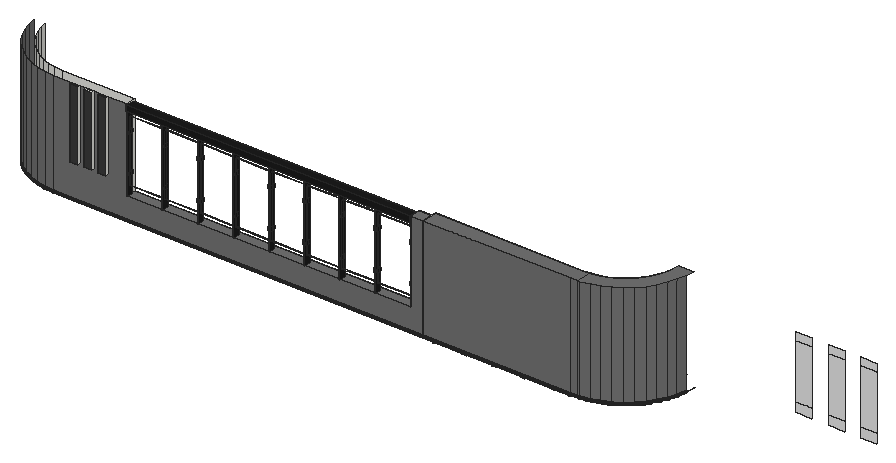
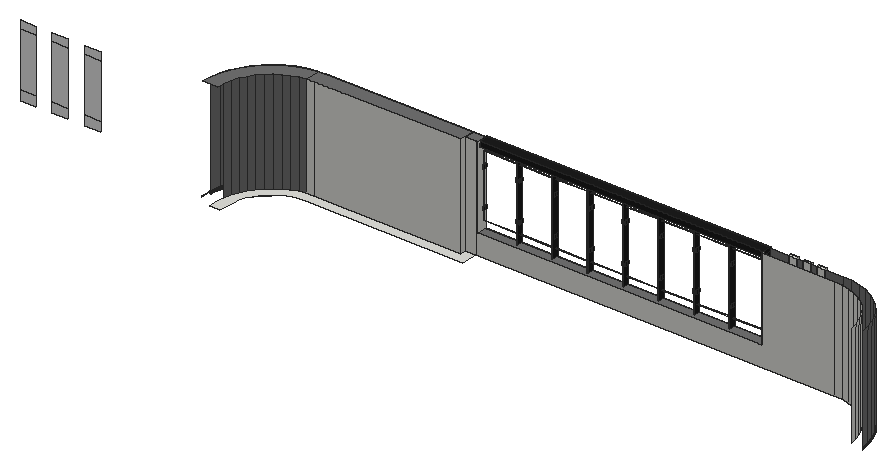
# SketchUp Ruby script. Lengths in inches.
U = 1.inch
M = Sketchup.active_model
def pt(a) = Geom::Point3d.new(a.map { |v| v * U })
def face(e, loops, mat)
  f = e.add_face(loops[0].map { |a| pt(a) })
  loops[1..].each { |l| e.add_face(l.map { |a| pt(a) }).erase! }
  f.material = f.back_material = mat if mat
  f
end
# faces: each face lists its corners as indices into pts; further lists are holes
def faces(e, pts, list, mat = nil) = list.each { |f| face(e, (f[0].is_a?(Array) ? f : [f]).map { |l| l.map { |i| pts[i] } }, mat) }
# xy, xz, yz: faces in a plane at the given z, y or x. An outline is a flat list of corners, or four numbers for a rectangle; further outlines are holes
def ring(l) = l.size == 4 ? [[l[0], l[1]], [l[2], l[1]], [l[2], l[3]], [l[0], l[3]]] : l.each_slice(2).to_a
def flat(e, list, mat, &to3) = list.each { |f| face(e, (f[0].is_a?(Array) ? f : [f]).map { |l| ring(l).map { |u, v| to3.(u, v) } }, mat) }
def xy(e, z, list, mat = nil) = flat(e, list, mat) { |x, y| [x, y, z] }
def xz(e, y, list, mat = nil) = flat(e, list, mat) { |x, z| [x, y, z] }
def yz(e, x, list, mat = nil) = flat(e, list, mat) { |y, z| [x, y, z] }
def lines(e, pts, list) = list.each { |a, b| e.add_line(pt(pts[a]), pt(pts[b])) }
# prism: a flat outline (further loops are holes) pulled along v
def prism(e, loops, v, mat = nil)
  f = face(e, loops, mat); d = Geom::Vector3d.new(v.map { |x| x * U })
  f.pushpull(f.normal.samedirection?(d) ? d.length : -d.length)
end
def box(e, o, s, mat = nil) = prism(e, [[o, [o[0] + s[0], o[1], o[2]], [o[0] + s[0], o[1] + s[1], o[2]], [o[0], o[1] + s[1], o[2]]]], [0, 0, s[2]], mat)
def at(x, y, z, deg = 0) = Geom::Transformation.translation(pt([x, y, z])) * Geom::Transformation.rotation(ORIGIN, Z_AXIS, deg.degrees)
def axes(o, x, y, z) = Geom::Transformation.new([*x, 0, *y, 0, *z, 0, *pt(o).to_a, 1])
def part(name) = M.definitions.add(name)
# library, detail: a bought-in or finely detailed component or shape, given as its bounding box
def library(name, o, s) = part(name).tap { |d| box(d.entities, o, s) }
def detail(e, o, s) = box(e.add_group.entities, o, s)
def put(e, d, t, mat = nil) = e.add_instance(d, t).tap { |i| i.material = mat if mat }
def group(e, t, mat = nil) = e.add_group.tap { |g| g.transformation = t; g.material = mat if mat }.entities
root = M.entities
M.materials.add("[0131_Silver]").color = [28, 28, 28]
M.materials.add("[Color M01]").color = [226, 226, 226]
M.materials.add("[Color M05]").color = [114, 114, 114]
M.materials.add("[Color M07]").color = [58, 58, 58]
M.materials.add("[Translucent_Glass_Blue]").color = [255, 255, 255]
M.materials["[Translucent_Glass_Blue]"].alpha = 0
c1 = part("Group\#11")
xy(c1.entities,0,[[0,0,0.39,2.125]],"[0131_Silver]")
xy(c1.entities,1.5,[[0,0,0.39,2.125]],"[0131_Silver]")
xz(c1.entities,0,[[0,0,0.39,1.5]],"[0131_Silver]")
xz(c1.entities,2.125,[[0,0,0.39,1.5]],"[0131_Silver]")
yz(c1.entities,0,[[0,0,2.125,1.5]],"[0131_Silver]")
yz(c1.entities,0.39,[[0,0,2.125,1.5]],"[0131_Silver]")
c2 = part("Glass railing panel")
xy(c2.entities,0,[[-0.59,0,0,63.98]])
xy(c2.entities,37.71,[[-0.59,0,0,63.98]])
xz(c2.entities,0,[[-0.59,0,0,37.71]])
xz(c2.entities,63.98,[[-0.59,0,0,37.71]])
yz(c2.entities,-0.59,[[0,0,63.98,37.71]])
yz(c2.entities,0,[[0,0,63.98,0,63.98,37.71,0,37.71,0,30.53,1.75,30.53,1.75,28.71,0,28.71],[-0.4,28.71,0,30.53],[0,28.71,1.75,30.53]])
p = [[0,63.98,30.53],[0.39,63.98,30.53]]
lines(c2.entities,p,[[0,1]])
put(c2.entities,c1,axes([0,62.22,28.71],[1,0,0],[0,1.01246,0],[0,0,1.2158]))
put(c2.entities,c1,axes([0,62.22,6.27],[1,0,0],[0,1.01246,0],[0,0,1.2158]))
put(c2.entities,c1,axes([0,0.6,28.71],[1,0,0],[0,1.01246,0],[0,0,1.2158]))
put(c2.entities,c1,axes([0,0.6,6.27],[1,0,0],[0,1.01246,0],[0,0,1.2158]))
put(c2.entities,c1,axes([-0.98,0.6,28.71],[1,0,0],[0,1.01246,0],[0,0,1.2158]))
put(c2.entities,c1,axes([-0.98,62.22,6.27],[1,0,0],[0,1.01246,0],[0,0,1.2158]))
put(c2.entities,c1,axes([-0.98,0.6,6.27],[1,0,0],[0,1.01246,0],[0,0,1.2158]))
put(c2.entities,c1,axes([-0.98,62.22,28.71],[1,0,0],[0,1.01246,0],[0,0,1.2158]))
c3 = part("Group\#1")
xz(c3.entities,0,[[0,0,1.97,38.58]])
xz(c3.entities,1.97,[[0,0,1.97,38.58]])
yz(c3.entities,0,[[0,0,1.97,37.71]])
yz(c3.entities,1.97,[[0,0,1.97,37.71]])
c4 = part("Glass railing section")
xy(c4.entities,37.71,[[2.51,0,3.15,0.39,3.15,0]])
xy(c4.entities,37.71,[[0,0,0.54,520.67],[2.51,0,2.51,63.58,3.15,0.39],[3.15,0.39,2.51,63.58,2.51,520.67,3.15,520.67]],"[0131_Silver]")
xy(c4.entities,38.58,[[0.54,496.0625,2.51,520.67]])
xy(c4.entities,38.58,[[0.54,0,2.51,496.0625]],"[0131_Silver]")
xy(c4.entities,40.46,[[0,0,3.15,520.67]],"[0131_Silver]")
xz(c4.entities,0,[[0,37.71,0.54,37.71,0.54,38.58,2.51,38.58,2.51,37.71,3.15,37.71,3.15,40.46,0,40.46]],"[0131_Silver]")
xz(c4.entities,520.67,[[0,37.71,0,40.46,3.15,40.46,3.15,37.71,2.51,37.71,2.51,38.58,0.54,38.58,0.54,37.71]])
yz(c4.entities,0,[[0,37.71,520.67,40.46]],"[0131_Silver]")
yz(c4.entities,0.54,[[496.0625,37.71,520.67,38.58]])
yz(c4.entities,0.54,[[0,37.71,496.0625,38.58]],"[0131_Silver]")
yz(c4.entities,2.51,[[0,37.71,496.0625,38.58],[496.0625,37.71,520.67,38.58]])
yz(c4.entities,3.15,[[0,37.71,520.67,40.46]],"[0131_Silver]")
put(c4.entities,c2,axes([1.8,65.35,3.9375],[1,0,0],[0,0.98769,0],[0,0,0.8225]),"[Translucent_Glass_Blue]")
put(c4.entities,c2,axes([1.8,130.31,3.9375],[1,0,0],[0,0.98769,0],[0,0,0.8225]),"[Translucent_Glass_Blue]")
put(c4.entities,c2,axes([1.8,195.28,3.9375],[1,0,0],[0,0.98769,0],[0,0,0.8225]),"[Translucent_Glass_Blue]")
put(c4.entities,c2,axes([1.8,260.24,3.9375],[1,0,0],[0,0.98769,0],[0,0,0.8225]),"[Translucent_Glass_Blue]")
put(c4.entities,c2,axes([1.8,325.2,3.9375],[1,0,0],[0,0.98769,0],[0,0,0.8225]),"[Translucent_Glass_Blue]")
put(c4.entities,c2,axes([1.8,390.16,3.9375],[1,0,0],[0,0.98769,0],[0,0,0.8225]),"[Translucent_Glass_Blue]")
put(c4.entities,c2,axes([1.8,455.12,3.9375],[1,0,0],[0,0.98769,0],[0,0,0.8225]),"[Translucent_Glass_Blue]")
put(c4.entities,c2,axes([1.8,0.39,3.9375],[1,0,0],[0,0.98769,0],[0,0,0.8225]),"[Translucent_Glass_Blue]")
put(c4.entities,c3,at(0.54,128.9375,0),"[0131_Silver]")
g1 = group(c4.entities,at(0.54,63.98,0),"[0131_Silver]")
xz(g1,0,[[0,0,1.97,38.58]])
xz(g1,1.97,[[0,0,1.97,38.58]])
yz(g1,0,[[0,0,1.97,37.71]])
yz(g1,1.97,[[0,0,1.97,37.71]])
put(c4.entities,c3,at(0.54,193.9,0),"[0131_Silver]")
put(c4.entities,c3,at(0.54,258.86,0),"[0131_Silver]")
put(c4.entities,c3,at(0.54,323.82,0),"[0131_Silver]")
put(c4.entities,c3,at(0.54,388.78,0),"[0131_Silver]")
put(c4.entities,c3,at(0.54,453.74,0),"[0131_Silver]")
put(c4.entities,c3,at(0.54,518.7,0),"[0131_Silver]")
c5 = part("Glass+Railing")
put(c5.entities,c4,axes([0,0,0],[1,0,0],[0,0.95652,0],[0,0,1]),"[0131_Silver]")
xy(root,251.12,[[157.86,0.53,159.39,0.93],[168.11,0.53,169.64,0.93],[178.36,0.53,179.89,0.93],[188.61,0.53,190.14,0.93],[198.86,0.53,200.39,0.93]])
xy(root,252,[[150.375,4.65,154.02,4.65,154.02,6.39,205.875,6.39,208.3,6.55,210.69,7.03,213,7.81,215.18,8.88,217.2,10.24,219.03,11.84,220.64,13.67,221.99,15.7,223.07,17.88,223.85,20.18,224.32,22.57,224.48,25,224.48,28.65,221.07,28.65,220.7,23.05,220.32,21.13,219.69,19.28,218.83,17.52,217.74,15.9,216.45,14.42,214.98,13.13,213.35,12.05,211.6,11.18,209.75,10.55,207.83,10.17,205.76,10.04,150.375,10.04]])
xy(root,259.1875,[[49.81,1,149.56,4.65]],"[Color M05]")
xy(root,263.625,[[30.59,0,33.34,1],[35.53,0,38.28,1],[40.47,0,43.22,1]])
xy(root,288,[[30.59,0,33.34,1],[35.53,0,38.28,1],[40.47,0,43.22,1]])
xy(root,288,[[149.56,1,154.02,4.65],[154.02,1,205.875,1,208.3,1.16,208.3,6.55,205.875,6.39,154.02,6.39],[208.3,1.16,209.01,1.21,212.09,1.82,215.06,2.83,217.875,4.22,220.49,5.96,222.85,8.03,224.92,10.39,226.66,13,228.05,15.82,229.06,18.79,229.67,21.87,229.875,25,224.48,25,224.32,22.57,223.85,20.18,223.07,17.88,221.99,15.7,220.64,13.67,219.03,11.84,217.2,10.24,215.18,8.88,213,7.81,210.69,7.03,208.3,6.55]],"[Color M05]")
xz(root,0,[[30.59,263.625,33.34,288],[35.53,263.625,38.28,288],[40.47,263.625,43.22,288]],"[Color M07]")
xz(root,1,[[30.59,263.625,33.34,288],[35.53,263.625,38.28,288],[40.47,263.625,43.22,288]])
xz(root,1,[[24.25,252,154.02,252,154.02,288,149.56,288,149.56,259.1875,49.81,259.1875,49.81,288,43.22,288,43.22,263.625,40.47,263.625,40.47,288,38.28,288,38.28,263.625,35.53,263.625,35.53,288,33.34,288,33.34,263.625,30.59,263.625,30.59,288,24.25,288],[154.02,252,205.875,288]],"[Color M05]")
xz(root,4.65,[[24.37,252,24.37,288,49.81,288,49.81,259.1875,149.56,259.1875,149.56,288,150.375,288,150.375,252],[150.375,252,154.02,288]])
xz(root,6.39,[[154.02,252,205.875,288]])
xz(root,23,[[267.39,257.79,273.02,261.06],[279.08,257.79,284.71,261.06],[290.02,257.79,295.64,261.06],[267.39,261.06,273.02,280.31],[279.08,261.06,284.71,280.31],
  [290.02,261.06,295.64,280.31],[267.39,280.31,273.02,283.04],[279.08,280.31,284.71,283.04],[290.02,280.31,295.64,283.04]],"[Color M01]")
yz(root,30.59,[[0,263.625,1,288]])
yz(root,33.34,[[0,263.625,1,288]])
yz(root,35.53,[[0,263.625,1,288]])
yz(root,38.28,[[0,263.625,1,288]])
yz(root,40.47,[[0,263.625,1,288]])
yz(root,43.22,[[0,263.625,1,288]])
yz(root,49.81,[[1,259.1875,4.65,288]])
yz(root,149.56,[[1,259.1875,4.65,288]])
yz(root,154.02,[[1,252,4.65,288],[4.65,252,6.39,288]])
p = [[21.1,1.07,251.1875],[21.11,1.13,251.12],[24.25,0.93,251.12],[24.25,0.87,251.1875],[21.12,1.21,251.0625],[24.25,1,251.0625],
  [154.02,0.93,251.12],[157.86,0.93,251.12],[159.39,0.93,251.12],[168.11,0.93,251.12],[169.64,0.93,251.12],[178.36,0.93,251.12],
  [179.89,0.93,251.12],[188.61,0.93,251.12],[190.14,0.93,251.12],[198.86,0.93,251.12],[200.39,0.93,251.12],[205.88,0.93,251.12],
  [205.88,0.87,251.1875],[154.02,0.87,251.1875],[154.02,1,251.0625],[205.875,1,251.0625],[208.31,1.09,251.12],[209.02,1.13,251.12],
  [209.03,1.07,251.1875],[208.3125,1.03,251.1875],[208.3,1.16,251.0625],[209.01,1.21,251.0625],[18,1.6875,251.1875],[18.02,1.75,251.12],
  [18.04,1.82,251.0625],[212.11,1.75,251.12],[212.12,1.6875,251.1875],[212.09,1.82,251.0625],[15.01,2.7,251.1875],[15.04,2.76,251.12],
  [15.07,2.83,251.0625],[215.09,2.76,251.12],[215.11,2.7,251.1875],[215.06,2.83,251.0625],[12.18,4.1,251.1875],[12.21,4.15,251.12],
  [217.91,4.15,251.12],[217.94,4.1,251.1875],[12.25,4.22,251.0625],[217.875,4.22,251.0625],[9.56,5.85,251.1875],[9.6,5.9,251.12],
  [220.53,5.9,251.12],[220.57,5.85,251.1875],[9.64,5.96,251.0625],[220.49,5.96,251.0625],[7.18,7.93,251.1875],[7.23,7.98,251.12],
  [7.28,8.03,251.0625],[222.9,7.98,251.12],[222.94,7.93,251.1875],[222.85,8.03,251.0625],[5.1,10.31,251.1875],[5.15,10.35,251.12],
  [224.97,10.35,251.12],[225.02,10.31,251.1875],[5.21,10.39,251.0625],[224.92,10.39,251.0625],[3.35,12.93,251.1875],[3.4,12.96,251.12],
  [3.47,13,251.0625],[226.66,13,251.0625],[226.72,12.96,251.12],[226.78,12.93,251.1875],[1.95,15.76,251.1875],[2.01,15.79,251.12],
  [228.11,15.79,251.12],[228.17,15.76,251.1875],[2.08,15.82,251.0625],[228.05,15.82,251.0625],[0.9375,18.75,251.1875],[1,18.77,251.12],
  [1.07,18.79,251.0625],[229.06,18.79,251.0625],[229.125,18.77,251.12],[229.1875,18.75,251.1875],[0.32,21.85,251.1875],[0.38,21.86,251.12],
  [0.46,21.87,251.0625],[229.74,21.86,251.12],[229.8,21.85,251.1875],[229.67,21.87,251.0625],[21.09,1.02,251.27],[24.24,0.82,251.27],
  [205.88,0.82,251.27],[154.02,0.82,251.27],[209.03,1.02,251.27],[208.32,0.98,251.27],[17.99,1.64,251.27],[212.13,1.64,251.27],
  [15,2.66,251.27],[215.13,2.66,251.27],[12.16,4.06,251.27],[217.97,4.06,251.27],[9.53,5.8125,251.27],[220.6,5.8125,251.27],
  [7.15,7.9,251.27],[222.98,7.9,251.27],[5.0625,10.28,251.27],[225.0625,10.28,251.27],[3.31,12.91,251.27],[226.82,12.91,251.27],
  [1.91,15.75,251.27],[228.22,15.75,251.27],[0.89,18.74,251.27],[229.23,18.74,251.27],[0.27,21.84,251.27],[229.85,21.84,251.27],
  [21.09,0.99,251.35],[24.24,0.78,251.35],[205.88,0.78,251.35],[154.02,0.78,251.35],[209.04,0.99,251.35],[208.32,0.94,251.35],
  [17.98,1.6,251.35],[212.14,1.6,251.35],[14.98,2.625,251.35],[215.14,2.625,251.35],[12.14,4.02,251.35],[217.99,4.02,251.35],
  [9.51,5.78,251.35],[220.62,5.78,251.35],[7.125,7.875,251.35],[223,7.875,251.35],[5.03,10.26,251.35],[225.09,10.26,251.35],
  [3.27,12.89,251.35],[226.85,12.89,251.35],[1.875,15.73,251.35],[228.25,15.73,251.35],[0.85,18.73,251.35],[229.27,18.73,251.35],
  [0.24,21.84,251.35],[229.89,21.84,251.35],[21.08,0.96,251.53],[21.09,0.96,251.4375],[24.24,0.76,251.4375],[24.24,0.75,251.53],
  [154.02,0.76,251.4375],[205.88,0.76,251.4375],[205.88,0.75,251.53],[154.02,0.75,251.53],[208.32,0.92,251.4375],[209.04,0.96,251.4375],
  [209.04,0.96,251.53],[208.32,0.91,251.53],[17.97,1.58,251.53],[17.98,1.58,251.4375],[212.15,1.58,251.4375],[212.15,1.58,251.53],
  [14.97,2.6,251.53],[14.97,2.6,251.4375],[215.15,2.6,251.4375],[215.16,2.6,251.53],[12.125,4,251.53],[12.13,4,251.4375],
  [218,4,251.4375],[218,4,251.53],[9.49,5.76,251.53],[9.49,5.77,251.4375],[220.63,5.77,251.4375],[220.64,5.76,251.53],
  [7.1,7.85,251.53],[7.11,7.86,251.4375],[223.02,7.86,251.4375],[223.02,7.85,251.53],[5.01,10.24,251.53],[5.02,10.24,251.4375],
  [225.11,10.24,251.4375],[225.11,10.24,251.53],[3.25,12.875,251.53],[3.25,12.88,251.4375],[226.87,12.88,251.4375],[226.875,12.875,251.53],
  [1.85,15.72,251.53],[1.85,15.72,251.4375],[228.27,15.72,251.4375],[228.28,15.72,251.53],[0.83,18.72,251.53],[0.83,18.73,251.4375],
  [229.29,18.73,251.4375],[229.3,18.72,251.53],[0.21,21.83,251.53],[0.21,21.84,251.4375],[229.91,21.84,251.4375],[229.92,21.83,251.53],
  [230.12,24.98,251.4375],[230.125,24.98,251.53],[21.09,0.96,251.625],[24.24,0.76,251.625],[205.88,0.76,251.625],[154.02,0.76,251.625],
  [209.04,0.96,251.625],[208.32,0.92,251.625],[17.98,1.58,251.625],[212.15,1.58,251.625],[14.97,2.6,251.625],[215.15,2.6,251.625],
  [12.13,4,251.625],[218,4,251.625],[9.49,5.77,251.625],[220.63,5.77,251.625],[7.11,7.86,251.625],[223.02,7.86,251.625],
  [5.02,10.24,251.625],[225.11,10.24,251.625],[3.25,12.88,251.625],[226.87,12.88,251.625],[1.85,15.72,251.625],[228.27,15.72,251.625],
  [0.83,18.73,251.625],[229.29,18.73,251.625],[0.21,21.84,251.625],[229.91,21.84,251.625],[230.12,24.98,251.625],[21.09,0.99,251.71],
  [24.24,0.78,251.71],[205.88,0.78,251.71],[154.02,0.78,251.71],[209.04,0.99,251.71],[208.32,0.94,251.71],[17.98,1.6,251.71],
  [212.14,1.6,251.71],[14.98,2.625,251.71],[215.14,2.625,251.71],[12.14,4.02,251.71],[217.99,4.02,251.71],[9.51,5.78,251.71],
  [220.62,5.78,251.71],[7.125,7.875,251.71],[223,7.875,251.71],[5.03,10.26,251.71],[225.09,10.26,251.71],[3.27,12.89,251.71],
  [226.85,12.89,251.71],[1.875,15.73,251.71],[228.25,15.73,251.71],[0.85,18.73,251.71],[229.27,18.73,251.71],[0.24,21.84,251.71],
  [229.89,21.84,251.71],[21.09,1.02,251.8],[24.24,0.82,251.8],[205.88,0.82,251.8],[154.02,0.82,251.8],[209.03,1.02,251.8],
  [208.32,0.98,251.8],[17.99,1.64,251.8],[212.13,1.64,251.8],[15,2.66,251.8],[215.13,2.66,251.8],[12.16,4.06,251.8],
  [217.97,4.06,251.8],[9.53,5.8125,251.8],[220.6,5.8125,251.8],[7.15,7.9,251.8],[222.98,7.9,251.8],[5.0625,10.28,251.8],
  [225.0625,10.28,251.8],[3.31,12.91,251.8],[226.82,12.91,251.8],[1.91,15.75,251.8],[228.22,15.75,251.8],[0.89,18.74,251.8],
  [229.23,18.74,251.8],[0.27,21.84,251.8],[229.85,21.84,251.8],[21.1,1.07,251.875],[24.25,0.87,251.875],[205.88,0.87,251.875],
  [154.02,0.87,251.875],[209.03,1.07,251.875],[208.3125,1.03,251.875],[18,1.6875,251.875],[212.12,1.6875,251.875],[15.01,2.7,251.875],
  [215.11,2.7,251.875],[12.18,4.1,251.875],[217.94,4.1,251.875],[9.56,5.85,251.875],[220.57,5.85,251.875],[7.18,7.93,251.875],
  [222.94,7.93,251.875],[5.1,10.31,251.875],[225.02,10.31,251.875],[3.35,12.93,251.875],[226.78,12.93,251.875],[1.95,15.76,251.875],
  [228.17,15.76,251.875],[0.9375,18.75,251.875],[229.1875,18.75,251.875],[0.32,21.85,251.875],[229.8,21.85,251.875],[21.11,1.13,251.94],
  [24.25,0.93,251.94],[21.12,1.21,252],[24.25,1,252],[205.88,0.93,251.94],[154.02,0.93,251.94],[205.875,1,252],
  [154.02,1,252],[209.02,1.13,251.94],[208.31,1.09,251.94],[209.01,1.21,252],[208.3,1.16,252],[18.02,1.75,251.94],
  [18.04,1.82,252],[212.11,1.75,251.94],[212.09,1.82,252],[15.04,2.76,251.94],[15.07,2.83,252],[215.09,2.76,251.94],
  [215.06,2.83,252],[12.21,4.15,251.94],[217.91,4.15,251.94],[12.25,4.22,252],[217.875,4.22,252],[9.6,5.9,251.94],
  [220.53,5.9,251.94],[9.64,5.96,252],[220.49,5.96,252],[7.23,7.98,251.94],[7.28,8.03,252],[222.9,7.98,251.94],
  [222.85,8.03,252],[5.15,10.35,251.94],[224.97,10.35,251.94],[5.21,10.39,252],[224.92,10.39,252],[3.4,12.96,251.94],
  [3.47,13,252],[226.72,12.96,251.94],[226.66,13,252],[2.01,15.79,251.94],[228.11,15.79,251.94],[2.08,15.82,252],
  [228.05,15.82,252],[1,18.77,251.94],[1.07,18.79,252],[229.125,18.77,251.94],[229.06,18.79,252],[0.38,21.86,251.94],
  [0.46,21.87,252],[229.74,21.86,251.94],[229.67,21.87,252],[24.25,1,288],[21.12,1.21,288],[208.3,1.16,288],
  [205.875,1,288],[18.04,1.82,288],[209.01,1.21,288],[212.09,1.82,288],[15.07,2.83,288],[215.06,2.83,288],
  [12.25,4.22,288],[217.875,4.22,288],[9.64,5.96,288],[220.49,5.96,288],[24.37,4.65,252],[21.59,4.83,252],
  [21.59,4.83,288],[24.37,4.65,288],[18.98,5.35,252],[18.98,5.35,288],[16.46,6.2,252],[16.46,6.2,288],
  [7.28,8.03,288],[222.85,8.03,288],[14.08,7.38,252],[14.08,7.38,288],[208.3,6.55,252],[205.875,6.39,252],
  [205.875,6.39,288],[208.3,6.55,288],[210.69,7.03,252],[210.69,7.03,288],[213,7.81,252],[213,7.81,288],
  [11.86,8.86,252],[11.86,8.86,288],[215.18,8.88,252],[215.18,8.88,288],[5.21,10.39,288],[224.92,10.39,288],
  [9.86,10.61,252],[9.86,10.61,288],[217.2,10.24,252],[217.2,10.24,288],[219.03,11.84,252],[219.03,11.84,288],
  [3.47,13,288],[226.66,13,288],[8.11,12.61,252],[8.11,12.61,288],[220.64,13.67,252],[220.64,13.67,288],
  [6.63,14.83,252],[6.63,14.83,288],[2.08,15.82,288],[228.05,15.82,288],[221.99,15.7,252],[221.99,15.7,288],
  [5.45,17.21,252],[5.45,17.21,288],[223.07,17.88,252],[223.07,17.88,288],[1.07,18.79,288],[229.06,18.79,288],
  [4.6,19.73,252],[4.6,19.73,288],[223.85,20.18,252],[223.85,20.18,288],[0.46,21.87,288],[229.67,21.87,288],
  [4.08,22.34,252],[4.08,22.34,288],[224.32,22.57,252],[224.32,22.57,288],[208.2,6.6875,251.4],[210.49,7.28,250.9],
  [212.71,8.14,250.5],[214.83,9.28,250.21],[216.8,10.66,250.03],[218.61,12.26,249.98],[220.22,14.07,250.03],[221.6,16.05,250.21],
  [222.73,18.16,250.5],[223.6,20.39,250.9],[224.1875,22.68,251.4]]
faces(root,p,[[0,1,2,3],[1,4,5,2],[3,2,6,7,8,9,10,11,12,13,14,15,16,17,18,19],[20,21,17,16,15,14,13,12,11,10,9,8,7,6,2,5],[18,17,22,23,24,25],[26,27,23,22,17,21],[28,29,1,0],[29,30,4,1],
  [24,23,31,32],[23,27,33,31],[34,35,29,28],[35,36,30,29],[32,31,37,38],[31,33,39,37],[40,41,35,34],[38,37,42,43],
  [41,44,36,35],[37,39,45,42],[46,47,41,40],[43,42,48,49],[47,50,44,41],[42,45,51,48],[52,53,47,46],[53,54,50,47],
  [49,48,55,56],[48,51,57,55],[58,59,53,52],[56,55,60,61],[59,62,54,53],[55,57,63,60],[64,65,59,58],[65,66,62,59],
  [60,63,67,68],[61,60,68,69],[70,71,65,64],[69,68,72,73],[71,74,66,65],[68,67,75,72],[76,77,71,70],[77,78,74,71],
  [72,75,79,80],[73,72,80,81],[82,83,77,76],[83,84,78,77],[81,80,85,86],[80,79,87,85],[88,0,3,89],[19,18,90,91,89,3],
  [90,18,25,24,92,93],[94,28,0,88],[92,24,32,95],[96,34,28,94],[95,32,38,97],[98,40,34,96],[97,38,43,99],[100,46,40,98],
  [99,43,49,101],[102,52,46,100],[101,49,56,103],[104,58,52,102],[103,56,61,105],[106,64,58,104],[105,61,69,107],[108,70,64,106],
  [107,69,73,109],[110,76,70,108],[109,73,81,111],[112,82,76,110],[111,81,86,113],[114,88,89,115],[91,90,116,117,115,89],[116,90,93,92,118,119],
  [120,94,88,114],[118,92,95,121],[122,96,94,120],[121,95,97,123],[124,98,96,122],[123,97,99,125],[126,100,98,124],[125,99,101,127],
  [128,102,100,126],[127,101,103,129],[130,104,102,128],[129,103,105,131],[132,106,104,130],[131,105,107,133],[134,108,106,132],[133,107,109,135],
  [136,110,108,134],[135,109,111,137],[138,112,110,136],[137,111,113,139],[140,141,142,143],[141,114,115,142],[143,142,144,145,146,147],[142,115,117,116,145,144],
  [146,145,148,149,150,151],[145,116,119,118,149,148],[152,153,141,140],[153,120,114,141],[150,149,154,155],[149,118,121,154],[156,157,153,152],[157,122,120,153],
  [155,154,158,159],[154,121,123,158],[160,161,157,156],[161,124,122,157],[158,123,125,162],[159,158,162,163],[164,165,161,160],[165,126,124,161],
  [163,162,166,167],[162,125,127,166],[168,169,165,164],[169,128,126,165],[167,166,170,171],[166,127,129,170],[172,173,169,168],[173,130,128,169],
  [171,170,174,175],[170,129,131,174],[176,177,173,172],[177,132,130,173],[175,174,178,179],[174,131,133,178],[180,181,177,176],[181,134,132,177],
  [179,178,182,183],[178,133,135,182],[184,185,181,180],[185,136,134,181],[183,182,186,187],[182,135,137,186],[188,189,185,184],[189,138,136,185],
  [187,186,190,191],[186,137,139,190],[191,190,192,193],[194,140,143,195],[147,146,196,197,195,143],[196,146,151,150,198,199],[200,152,140,194],[198,150,155,201],
  [202,156,152,200],[201,155,159,203],[204,160,156,202],[203,159,163,205],[206,164,160,204],[205,163,167,207],[208,168,164,206],[207,167,171,209],
  [210,172,168,208],[209,171,175,211],[212,176,172,210],[211,175,179,213],[214,180,176,212],[213,179,183,215],[216,184,180,214],[215,183,187,217],
  [218,188,184,216],[217,187,191,219],[219,191,193,220],[221,194,195,222],[197,196,223,224,222,195],[223,196,199,198,225,226],[227,200,194,221],[225,198,201,228],
  [229,202,200,227],[228,201,203,230],[231,204,202,229],[230,203,205,232],[233,206,204,231],[232,205,207,234],[235,208,206,233],[234,207,209,236],
  [237,210,208,235],[236,209,211,238],[239,212,210,237],[238,211,213,240],[241,214,212,239],[240,213,215,242],[243,216,214,241],[242,215,217,244],
  [245,218,216,243],[244,217,219,246],[247,221,222,248],[224,223,249,250,248,222],[249,223,226,225,251,252],[253,227,221,247],[251,225,228,254],[255,229,227,253],
  [254,228,230,256],[257,231,229,255],[256,230,232,258],[259,233,231,257],[258,232,234,260],[261,235,233,259],[260,234,236,262],[263,237,235,261],
  [262,236,238,264],[265,239,237,263],[264,238,240,266],[267,241,239,265],[266,240,242,268],[269,243,241,267],[268,242,244,270],[271,245,243,269],
  [270,244,246,272],[273,247,248,274],[274,248,250,249,275,276],[275,249,252,251,277,278],[279,253,247,273],[277,251,254,280],[281,255,253,279],[280,254,256,282],
  [283,257,255,281],[282,256,258,284],[285,259,257,283],[284,258,260,286],[287,261,259,285],[286,260,262,288],[289,263,261,287],[288,262,264,290],
  [291,265,263,289],[290,264,266,292],[293,267,265,291],[292,266,268,294],[295,269,267,293],[294,268,270,296],[297,271,269,295],[296,270,272,298],
  [299,273,274,300],[301,299,300,302],[300,274,276,275,303,304],[304,303,305,306,302,300],[303,275,278,277,307,308],[305,303,308,307,309,310],[311,279,273,299],[312,311,299,301],
  [307,277,280,313],[309,307,313,314],[315,281,279,311],[316,315,311,312],[313,280,282,317],[314,313,317,318],[319,283,281,315],[317,282,284,320],
  [321,319,315,316],[318,317,320,322],[323,285,283,319],[320,284,286,324],[325,323,319,321],[322,320,324,326],[327,287,285,323],[328,327,323,325],
  [324,286,288,329],[326,324,329,330],[331,289,287,327],[329,288,290,332],[333,331,327,328],[330,329,332,334],[335,291,289,331],[336,335,331,333],
  [334,332,337,338],[332,290,292,337],[339,293,291,335],[337,292,294,340],[341,339,335,336],[338,337,340,342],[343,295,293,339],[344,343,339,341],
  [342,340,345,346],[340,294,296,345],[347,297,295,343],[348,347,343,344],[345,296,298,349],[346,345,349,350]],"[Color M07]")
faces(root,p,[[301,302,351,352],[305,310,353,354],[312,301,352,355],[310,309,356,353],[309,314,357,356],[316,312,355,358],[314,318,359,357],[321,316,358,360],
  [318,322,361,359],[325,321,360,362],[322,326,363,361],[328,325,362,372],[326,330,373,363],[380,376,379,381],[382,380,381,383],[386,382,383,387],
  [333,328,372,388],[330,334,389,373],[392,386,387,393],[394,392,393,395],[336,333,388,396],[334,338,397,389],[400,394,395,401],[341,336,396,404],
  [338,342,405,397],[406,400,401,407],[410,406,407,411],[344,341,404,412],[342,346,413,405],[416,410,411,417],[348,344,412,418],[346,350,419,413],
  [422,416,417,423]],"[Color M05]")
faces(root,p,[[364,365,366,367],[365,368,369,366],[368,370,371,369],[370,374,375,371],[376,377,378,379],[374,384,385,375],[384,390,391,385],[390,398,399,391],
  [398,402,403,399],[402,408,409,403],[408,414,415,409],[414,420,421,415]])
lines(root,p,[[377,424],[424,425],[425,426],[426,427],[427,428],[428,429],[429,430],[430,431],[431,432],[432,433],[433,434]])
put(root,c5,axes([149.56,0.46,259.1875],[0,1,0],[-0.20029,0,0],[0,0,0.71207]))
